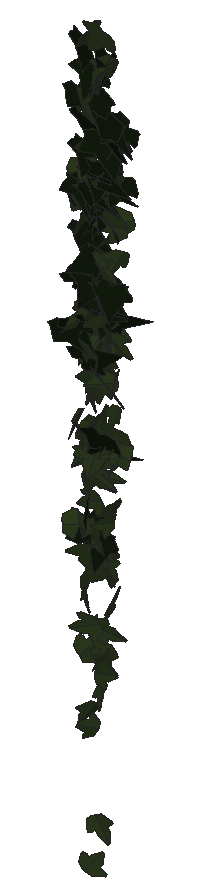
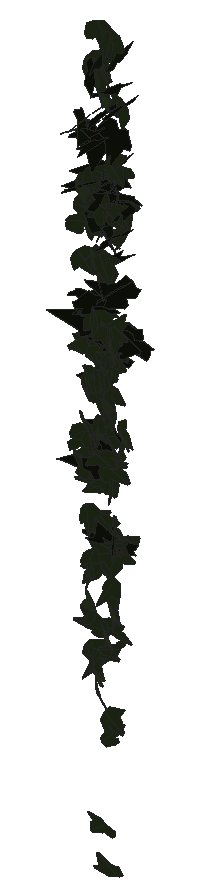
# SketchUp Ruby script. Lengths in inches.
U = 1.inch
M = Sketchup.active_model
def pt(a) = Geom::Point3d.new(a.map { |v| v * U })
def face(e, loops, mat)
  f = e.add_face(loops[0].map { |a| pt(a) })
  loops[1..].each { |l| e.add_face(l.map { |a| pt(a) }).erase! }
  f.material = f.back_material = mat if mat
  f
end
# faces: each face lists its corners as indices into pts; further lists are holes
def faces(e, pts, list, mat = nil) = list.each { |f| face(e, (f[0].is_a?(Array) ? f : [f]).map { |l| l.map { |i| pts[i] } }, mat) }
# xy, xz, yz: faces in a plane at the given z, y or x. An outline is a flat list of corners, or four numbers for a rectangle; further outlines are holes
def ring(l) = l.size == 4 ? [[l[0], l[1]], [l[2], l[1]], [l[2], l[3]], [l[0], l[3]]] : l.each_slice(2).to_a
def flat(e, list, mat, &to3) = list.each { |f| face(e, (f[0].is_a?(Array) ? f : [f]).map { |l| ring(l).map { |u, v| to3.(u, v) } }, mat) }
def xy(e, z, list, mat = nil) = flat(e, list, mat) { |x, y| [x, y, z] }
def xz(e, y, list, mat = nil) = flat(e, list, mat) { |x, z| [x, y, z] }
def yz(e, x, list, mat = nil) = flat(e, list, mat) { |y, z| [x, y, z] }
def lines(e, pts, list) = list.each { |a, b| e.add_line(pt(pts[a]), pt(pts[b])) }
# prism: a flat outline (further loops are holes) pulled along v
def prism(e, loops, v, mat = nil)
  f = face(e, loops, mat); d = Geom::Vector3d.new(v.map { |x| x * U })
  f.pushpull(f.normal.samedirection?(d) ? d.length : -d.length)
end
def box(e, o, s, mat = nil) = prism(e, [[o, [o[0] + s[0], o[1], o[2]], [o[0] + s[0], o[1] + s[1], o[2]], [o[0], o[1] + s[1], o[2]]]], [0, 0, s[2]], mat)
def at(x, y, z, deg = 0) = Geom::Transformation.translation(pt([x, y, z])) * Geom::Transformation.rotation(ORIGIN, Z_AXIS, deg.degrees)
def axes(o, x, y, z) = Geom::Transformation.new([*x, 0, *y, 0, *z, 0, *pt(o).to_a, 1])
def part(name) = M.definitions.add(name)
# library, detail: a bought-in or finely detailed component or shape, given as its bounding box
def library(name, o, s) = part(name).tap { |d| box(d.entities, o, s) }
def detail(e, o, s) = box(e.add_group.entities, o, s)
def put(e, d, t, mat = nil) = e.add_instance(d, t).tap { |i| i.material = mat if mat }
def group(e, t, mat = nil) = e.add_group.tap { |g| g.transformation = t; g.material = mat if mat }.entities
root = M.entities
M.materials.add("1026 AP 7946 SUNNY SIDE UP").color = [254, 231, 186]
M.materials.add("efeu1").color = [18, 25, 13]
M.materials.add("efeu2").color = [43, 57, 29]
c1 = part("ivyleaf_10")
p = [[0,0.5,-0.03],[-0.0625,2.02,-0.43],[-0.19,2.01,-0.46],[-0.54,1.05,-0.29],[-0.52,0.625,-0.18],[-0.83,0.76,-0.28],
  [-1.16,0.64,-0.33],[-1.15,0.33,-0.24],[-0.77,-0.39,0.02],[-0.3,-0.51,0.16],[0.04,-0.48,0.23],[-0.02,2.01,-0.4375],
  [-0.06,2.01,-0.43],[0.04,-0.49,0.23],[0.67,-0.49,0.14],[1.38,0.36,-0.2],[1.375,0.51,-0.24],[0.81,0.65,-0.19],
  [0.62,0.59,-0.15],[0.6,1.09,-0.28],[0.5,1.23,-0.31]]
faces(c1.entities,p,[[0,1,2,3,4,5,6,7,8,9,10],[11,12,0,13,14,15,16,17,18,19,20]],"efeu2")
c2 = part("ivyleaf_9")
p = [[1.54,2.16,1.25],[1.36,2.04,1.19],[-0.21,0.99,0.68],[-0.71,1.11,0.82],[-0.85,0.86,0.67],[-0.8,0.17,0.21],
  [-0.9,-0.01,0.1],[-0.67,-0.16,-0.02],[-0.08,-0.08,-0.05],[-0.03,-0.6,-0.4],[0.65,-0.88,-0.66],[0.83,-0.6,-0.49],
  [1.29,-0.42,-0.43],[1.8125,-0.07,-0.26],[1.21,0.44,0.15]]
faces(c2.entities,p,[[0,1,2,3,4,5,6,7,8,9,10,11,12,13,14]],"efeu1")
put(root,c1,axes([106.17,212.36,258.08],[-0.20733,0.18687,0.08375],[0.07494,-0.06456,0.23523],[0.31087,0.1402,-0.00085]),"1026 AP 7946 SUNNY SIDE UP")
put(root,c1,axes([106.34,212.28,263.92],[-0.33915,-0.0739,0.11531],[-0.15457,-0.05825,-0.23424],[0.14429,-0.23612,0.0201]),"1026 AP 7946 SUNNY SIDE UP")
put(root,c1,axes([106.14,212.3,258.68],[0.16961,-0.19678,0.12508],[0.06388,-0.11701,-0.23111],[0.35886,0.11384,-0.01798]),"1026 AP 7946 SUNNY SIDE UP")
put(root,c1,axes([106.21,212.55,264.98],[0.01795,-0.24608,0.10694],[0.02224,-0.10459,-0.25424],[0.42022,0.01604,0.00889]),"1026 AP 7946 SUNNY SIDE UP")
put(root,c2,axes([105.98,212.14,260.81],[-0.09391,-0.08738,-0.23628],[0.27532,0.14952,-0.10501],[0.2694,-0.18327,0.02496]),"1026 AP 7946 SUNNY SIDE UP")
put(root,c1,axes([106.36,212.21,256.09],[0.2074,-0.01936,0.18283],[-0.26065,0.06899,0.135],[-0.10466,-0.21017,0.0261]),"1026 AP 7946 SUNNY SIDE UP")
put(root,c1,axes([106.22,212.48,260.36],[-0.05254,-0.20434,-0.10501],[0.02558,0.09945,-0.21272],[0.35733,-0.03717,-0.00021]),"1026 AP 7946 SUNNY SIDE UP")
put(root,c1,axes([106,212.17,256.13],[0.08141,-0.06725,-0.23613],[0.29084,0.15915,-0.00414],[0.23677,-0.17237,0.08628]),"1026 AP 7946 SUNNY SIDE UP")
put(root,c1,axes([106.19,212.5,260.3125],[0.04478,0.16939,-0.1684],[-0.04149,-0.1623,-0.1779],[-0.36887,0.03882,-0.00043]),"1026 AP 7946 SUNNY SIDE UP")
put(root,c1,axes([106.22,212.53,254.72],[0.10449,-0.19811,0.05644],[0.0243,-0.05379,-0.21557],[0.32276,0.06818,-0.00204]),"1026 AP 7946 SUNNY SIDE UP")
put(root,c2,axes([106.21,212.36,265.67],[0.35397,-0.0276,-0.15543],[-0.24035,-0.02181,-0.23121],[0.01677,0.27003,-0.03295]),"1026 AP 7946 SUNNY SIDE UP")
put(root,c1,axes([106.32,212.6,263.89],[-0.17824,-0.15521,0.146],[-0.04027,-0.15058,-0.19069],[0.32897,-0.10253,0.05576]),"1026 AP 7946 SUNNY SIDE UP")
put(root,c1,axes([106.26,212.39,261.04],[-0.02348,-0.06015,0.26537],[0.02207,-0.25816,-0.0627],[0.41587,0.0103,0.01831]),"1026 AP 7946 SUNNY SIDE UP")
put(root,c1,axes([106.14,212.5,264.31],[-0.07374,0.08614,-0.22795],[0.08089,-0.217,-0.09932],[-0.36522,-0.06545,0.02403]),"1026 AP 7946 SUNNY SIDE UP")
put(root,c1,axes([106.29,212.1,263.15],[0.04385,-0.04155,0.25671],[-0.13514,0.23444,0.0515],[-0.37393,-0.0896,0.01149]),"1026 AP 7946 SUNNY SIDE UP")
put(root,c1,axes([106.39,212.53,256.66],[0.19892,-0.06102,-0.15531],[-0.21651,0.06065,-0.14429],[0.13517,0.18695,-0.00256]),"1026 AP 7946 SUNNY SIDE UP")
put(root,c2,axes([106.35,212.28,256.49],[0.06178,-0.04328,-0.24801],[-0.31387,0.13482,-0.0578],[0.22163,0.203,-0.01272]),"1026 AP 7946 SUNNY SIDE UP")
put(root,c1,axes([106.36,212.51,261.01],[-0.33357,-0.03615,0.06661],[-0.09204,-0.03942,-0.22007],[0.07186,-0.21831,0.02736]),"1026 AP 7946 SUNNY SIDE UP")
put(root,c2,axes([106,212.13,260.73],[0.16843,0.05581,0.23152],[0.33879,0.06573,-0.12241],[-0.13205,0.23982,-0.01874]),"1026 AP 7946 SUNNY SIDE UP")
put(root,c1,axes([106.25,212.46,260.69],[0.08806,-0.20288,0.09923],[0.05222,-0.0919,-0.21725],[0.35005,0.06475,0.00744]),"1026 AP 7946 SUNNY SIDE UP")
put(root,c1,axes([106.2,212.54,259.17],[-0.18005,0.15457,-0.08059],[0.06462,-0.06793,-0.19844],[-0.26526,-0.12146,0.00635]),"1026 AP 7946 SUNNY SIDE UP")
put(root,c1,axes([106.39,212.41,257.8125],[-0.13486,-0.12628,0.156],[-0.113,-0.13459,-0.15761],[0.28964,-0.11131,0.01114]),"1026 AP 7946 SUNNY SIDE UP")
put(root,c2,axes([106.1,212.35,266.28],[0.12046,-0.25366,-0.08776],[-0.02131,0.08332,-0.27227],[0.41949,0.07708,0.01137]),"1026 AP 7946 SUNNY SIDE UP")
put(root,c1,axes([106.24,212.68,259.55],[0.05685,-0.15964,0.15075],[0.08218,-0.13848,-0.16871],[0.33145,0.06171,0.01597]),"1026 AP 7946 SUNNY SIDE UP")
put(root,c2,axes([106.08,212.29,261.82],[0.00888,-0.00129,0.26076],[0.37397,0.0867,-0.0045],[-0.13625,0.23788,0.00464]),"1026 AP 7946 SUNNY SIDE UP")
put(root,c1,axes([106.37,212.21,254.52],[-0.14827,0.14765,0.13583],[-0.12718,0.10354,-0.17959],[-0.28313,-0.12383,0.00954]),"1026 AP 7946 SUNNY SIDE UP")
put(root,c2,axes([106.16,212.43,267.32],[-0.00258,-0.19972,0.18724],[0.00235,-0.18289,-0.20681],[0.42581,-0.0002,0.00228]),"1026 AP 7946 SUNNY SIDE UP")
put(root,c1,axes([106.29,212.6,259.29],[0.18601,-0.17829,0.03368],[0.01611,-0.03361,-0.22039],[0.28486,0.11832,-0.00953]),"1026 AP 7946 SUNNY SIDE UP")
put(root,c2,axes([106.21,212.45,264.84],[-0.0488,-0.20698,0.13975],[-0.00643,-0.13745,-0.21596],[0.39009,-0.02816,0.01392]),"1026 AP 7946 SUNNY SIDE UP")
put(root,c2,axes([106.29,212.62,266.7],[-0.15011,-0.2225,0.07101],[-0.01559,-0.07191,-0.24912],[0.36652,-0.09419,0.01849]),"1026 AP 7946 SUNNY SIDE UP")
put(root,c1,axes([106.19,212.46,258.29],[0.23853,-0.0907,0.1462],[0.16646,-0.09808,-0.18108],[0.20685,0.18352,-0.02287]),"1026 AP 7946 SUNNY SIDE UP")
put(root,c1,axes([106.36,212.125,260.48],[-0.29982,0.11659,0.00771],[-0.02687,-0.01494,-0.22925],[-0.18167,-0.19021,0.02119]),"1026 AP 7946 SUNNY SIDE UP")
put(root,c1,axes([106.16,212.27,266.16],[-0.17241,0.08051,-0.24277],[0.2305,-0.18789,-0.13723],[-0.31738,-0.18019,0.03221]),"1026 AP 7946 SUNNY SIDE UP")
put(root,c1,axes([106.38,212.36,267.72],[-0.07357,-0.23047,-0.16421],[0.05122,0.1547,-0.24136],[0.43645,-0.05701,0.00064]),"1026 AP 7946 SUNNY SIDE UP")
put(root,c1,axes([106.4375,212.64,258.17],[0.20828,0.11392,-0.13528],[-0.14482,-0.09499,-0.18027],[-0.23274,0.16105,-0.00889]),"1026 AP 7946 SUNNY SIDE UP")
put(root,c1,axes([106.44,212.59,262.68],[-0.10697,-0.21769,0.03991],[-0.00785,-0.0403,-0.23508],[0.34793,-0.06783,0.00697]),"1026 AP 7946 SUNNY SIDE UP")
put(root,c2,axes([106.31,212.35,264.14],[-0.22126,-0.18156,-0.11538],[0.15175,0.06412,-0.23376],[0.29819,-0.16734,0.03335]),"1026 AP 7946 SUNNY SIDE UP")
put(root,c1,axes([106.42,212.52,260.08],[0.01291,-0.21517,-0.06571],[0.01909,0.06294,-0.22099],[0.35182,0.00448,0.0144]),"1026 AP 7946 SUNNY SIDE UP")
put(root,c2,axes([106.37,212.42,261.85],[-0.11322,-0.21238,0.12841],[-0.04726,-0.12258,-0.23153],[0.38529,-0.07744,0.00933]),"1026 AP 7946 SUNNY SIDE UP")
put(root,c2,axes([106.24,212.29,263.19],[0.17485,-0.18056,-0.17361],[-0.04148,0.17399,-0.21024],[0.38503,0.10074,0.05619]),"1026 AP 7946 SUNNY SIDE UP")
put(root,c2,axes([106.4,212.33,263.83],[0.17196,-0.11205,-0.2086],[-0.24119,0.13166,-0.16013],[0.2713,0.18807,-0.01015]),"1026 AP 7946 SUNNY SIDE UP")
put(root,c1,axes([106.375,212.32,255.08],[-0.03474,-0.16013,-0.19442],[0.11748,0.17537,-0.16207],[0.36987,-0.07074,0.03322]),"1026 AP 7946 SUNNY SIDE UP")
put(root,c1,axes([106.49,212.28,251.97],[-0.03873,-0.19817,0.11264],[-0.02551,-0.10929,-0.20635],[0.35583,-0.02941,-0.00254]),"1026 AP 7946 SUNNY SIDE UP")
put(root,c1,axes([106.5,212.09,257.36],[-0.07802,0.15391,0.18517],[-0.14048,0.15692,-0.16372],[-0.34342,-0.09916,0.0249]),"1026 AP 7946 SUNNY SIDE UP")
put(root,c2,axes([106.22,212.36,264.01],[-0.02716,-0.07377,-0.25379],[0.17644,0.21953,-0.07468],[0.36313,-0.11218,0.0173]),"1026 AP 7946 SUNNY SIDE UP")
put(root,c1,axes([106.34,212.23,264.67],[0.31457,0.13701,0.02611],[0.04398,0.00257,-0.24938],[-0.2144,0.20154,-0.01284]),"1026 AP 7946 SUNNY SIDE UP")
put(root,c2,axes([106.41,212.6,263.41],[-0.25216,0.0307,-0.19145],[0.27551,-0.06586,-0.16721],[-0.10941,-0.2366,0.02019]),"1026 AP 7946 SUNNY SIDE UP")
put(root,c1,axes([106.16,212.58,260.33],[-0.00749,-0.01037,0.23903],[0.36441,0.01597,0.00573],[-0.02546,0.23158,0.01168]),"1026 AP 7946 SUNNY SIDE UP")
put(root,c1,axes([106.63,212.15,253.99],[0.19782,-0.0573,-0.17662],[-0.26579,0.03561,-0.1401],[0.09935,0.20938,-0.02316]),"1026 AP 7946 SUNNY SIDE UP")
put(root,c1,axes([106.57,212.53,259.49],[-0.26463,0.10457,0.07881],[-0.1461,-0.01133,-0.19623],[-0.14118,-0.18427,0.05535]),"1026 AP 7946 SUNNY SIDE UP")
put(root,c1,axes([106.375,212.625,266.59],[0.14064,-0.14966,0.1966],[0.14051,-0.16973,-0.18046],[0.35564,0.12624,-0.00645]),"1026 AP 7946 SUNNY SIDE UP")
put(root,c1,axes([106.49,212.37,259.58],[-0.39898,0.01824,-0.00673],[0.00735,-0.027,-0.2608],[-0.02963,-0.25238,0.02592]),"1026 AP 7946 SUNNY SIDE UP")
put(root,c1,axes([106.52,212.43,264.06],[0.16552,-0.13106,-0.17869],[-0.05801,0.17836,-0.16155],[0.33593,0.09538,0.06015]),"1026 AP 7946 SUNNY SIDE UP")
put(root,c2,axes([106.43,212.23,255.89],[-0.32401,0.03737,0.16518],[0.25087,-0.01663,0.21542],[0.06251,0.26043,-0.00839]),"1026 AP 7946 SUNNY SIDE UP")
put(root,c1,axes([106.39,212.35,260.27],[0.17732,0.11369,-0.15923],[0.11591,0.14064,0.16213],[0.27943,-0.13049,0.03379]),"1026 AP 7946 SUNNY SIDE UP")
put(root,c1,axes([106.53,212.2,255.7],[-0.31291,-0.17336,0.00168],[0.01718,-0.01651,-0.27123],[0.27208,-0.19833,0.01906]),"1026 AP 7946 SUNNY SIDE UP")
put(root,c2,axes([106.5625,212.38,262.42],[-0.15697,-0.12815,0.22117],[-0.17755,-0.18401,-0.16776],[0.35186,-0.15002,0.01401]),"1026 AP 7946 SUNNY SIDE UP")
put(root,c1,axes([106.51,212.31,251.47],[-0.00624,0.09865,0.19903],[0.01739,-0.19233,0.10057],[0.33987,0.01165,-0.00149]),"1026 AP 7946 SUNNY SIDE UP")
put(root,c2,axes([106.24,212.36,263.83],[0.24059,-0.17517,0.11175],[0.09539,-0.09212,-0.23975],[0.31048,0.16405,-0.01294]),"1026 AP 7946 SUNNY SIDE UP")
put(root,c1,axes([106.39,212.4,253.73],[0.09725,-0.12721,-0.15696],[0.13129,-0.12727,0.14433],[-0.28217,-0.10306,0.01306]),"1026 AP 7946 SUNNY SIDE UP")
put(root,c2,axes([106.41,212.57,266.12],[0.07787,-0.24413,-0.06587],[-0.03387,0.05942,-0.2561],[0.39482,0.05324,-0.00898]),"1026 AP 7946 SUNNY SIDE UP")
put(root,c1,axes([106.59,212.47,259.74],[-0.0163,-0.19104,0.12763],[0.00136,-0.12513,-0.19772],[0.35896,-0.0082,0.00654]),"1026 AP 7946 SUNNY SIDE UP")
put(root,c1,axes([106.6,212.6,262.77],[0.0614,-0.22971,0.02809],[0.00081,-0.02889,-0.24016],[0.36397,0.03881,-0.0042]),"1026 AP 7946 SUNNY SIDE UP")
put(root,c2,axes([106.46,212.51,264.39],[-0.05821,-0.23811,0.1155],[0.02215,-0.1162,-0.24716],[0.41416,-0.02725,0.02945]),"1026 AP 7946 SUNNY SIDE UP")
put(root,c1,axes([106.77,212.26,267.82],[-0.35601,0.05025,0.13611],[-0.21439,-0.01382,-0.23587],[-0.05706,-0.26163,0.03701]),"1026 AP 7946 SUNNY SIDE UP")
put(root,c1,axes([106.64,212.42,266.82],[0.05518,-0.27743,-0.09139],[-0.01821,0.08636,-0.28758],[0.45688,0.03695,-0.00042]),"1026 AP 7946 SUNNY SIDE UP")
put(root,c1,axes([106.5,211.99,253.4],[0.12518,0.05749,-0.226],[0.1403,0.20617,0.0901],[0.32837,-0.11,0.04766]),"1026 AP 7946 SUNNY SIDE UP")
put(root,c1,axes([106.61,212.48,258.79],[-0.00084,-0.19201,-0.10703],[0.02748,0.10243,-0.19659],[0.34135,-0.00872,0.01557]),"1026 AP 7946 SUNNY SIDE UP")
put(root,c2,axes([106.47,212.09,264.28],[0.24852,-0.13811,-0.15342],[-0.11925,0.13388,-0.21115],[0.29529,0.1703,0.04385]),"1026 AP 7946 SUNNY SIDE UP")
put(root,c1,axes([106.63,212.47,258.77],[0.0501,-0.20321,0.07242],[0.01001,-0.07131,-0.21227],[0.33856,0.03218,-0.00444]),"1026 AP 7946 SUNNY SIDE UP")
put(root,c1,axes([106.625,212.59,259.89],[0.00136,-0.19049,0.10999],[0.02761,-0.10744,-0.19627],[0.34309,0.0094,0.01536]),"1026 AP 7946 SUNNY SIDE UP")
put(root,c1,axes([106.65,212.4,262.2],[0.08522,-0.22582,-0.05665],[-0.01121,0.0535,-0.23887],[0.36482,0.05439,0.00589]),"1026 AP 7946 SUNNY SIDE UP")
put(root,c2,axes([106.81,212.65,261.52],[-0.07745,0.00611,0.25172],[-0.33851,-0.11903,-0.04234],[0.18186,-0.21896,0.02839]),"1026 AP 7946 SUNNY SIDE UP")
put(root,c1,axes([106.59,212.23,257.94],[0.37564,-0.00386,-0.01181],[-0.01845,-0.02079,-0.24531],[0.00448,0.23826,-0.02019]),"1026 AP 7946 SUNNY SIDE UP")
put(root,c2,axes([106.53,212.64,267.17],[-0.07894,-0.13575,0.22304],[0.00442,-0.22168,-0.14332],[0.40282,-0.02417,0.04528]),"1026 AP 7946 SUNNY SIDE UP")
put(root,c2,axes([106.75,212.375,263.59],[-0.15352,0.19218,-0.14327],[0.08688,-0.12904,-0.22268],[-0.36378,-0.11192,0.00728]),"1026 AP 7946 SUNNY SIDE UP")
put(root,c1,axes([106.4,212.32,258.53],[0.16658,0.00113,0.21861],[0.33355,-0.0067,-0.1091],[0.00863,0.23707,-0.00274]),"1026 AP 7946 SUNNY SIDE UP")
put(root,c1,axes([106.45,212.27,256],[0.1813,-0.03816,0.18675],[0.27625,-0.04598,-0.12521],[0.09341,0.21004,0.00785]),"1026 AP 7946 SUNNY SIDE UP")
put(root,c1,axes([106.58,212.45,260.34],[0.10253,-0.12774,0.18836],[0.15412,-0.15554,-0.14828],[0.31606,0.11728,0.01121]),"1026 AP 7946 SUNNY SIDE UP")
put(root,c1,axes([106.69,212.5,261.36],[0.02761,-0.20979,-0.09604],[0.02938,0.09331,-0.2149],[0.35903,0.0085,0.02497]),"1026 AP 7946 SUNNY SIDE UP")
put(root,c2,axes([106.4,212.14,260.125],[-0.0022,0.02724,0.25442],[0.34677,-0.11327,0.01351],[0.1794,0.21928,-0.02299]),"1026 AP 7946 SUNNY SIDE UP")
put(root,c1,axes([106.52,212.37,255.79],[-0.19592,0.02972,-0.16682],[0.22477,-0.08165,-0.12909],[-0.12897,-0.18744,0.02845]),"1026 AP 7946 SUNNY SIDE UP")
put(root,c1,axes([106.48,212.48,260.86],[-0.20299,0.03014,0.19826],[0.3052,0.00291,0.1338],[0.02259,0.23158,-0.02611]),"1026 AP 7946 SUNNY SIDE UP")
put(root,c1,axes([106.54,212.12,248.3],[0.2865,-0.03067,-0.09394],[0.14601,0.0064,0.18932],[-0.03858,-0.20357,0.01888]),"1026 AP 7946 SUNNY SIDE UP")
put(root,c1,axes([106.55,212.29,257.4],[-0.22426,-0.05792,-0.1559],[0.23419,0.03145,-0.15716],[0.09914,-0.20531,0.01858]),"1026 AP 7946 SUNNY SIDE UP")
put(root,c1,axes([106.64,212.47,253.05],[0.11553,-0.13936,0.14741],[0.0997,-0.12919,-0.16302],[0.29876,0.097,-0.0026]),"1026 AP 7946 SUNNY SIDE UP")
put(root,c1,axes([106.61,212.61,259.98],[-0.21649,0.10661,-0.12779],[0.12076,-0.1019,-0.17777],[-0.2279,-0.15527,0.02719]),"1026 AP 7946 SUNNY SIDE UP")
put(root,c1,axes([106.64,212.46,261.34],[-0.29982,-0.08425,-0.08348],[0.13932,-0.00441,-0.21134],[0.1191,-0.20694,0.03708]),"1026 AP 7946 SUNNY SIDE UP")
put(root,c1,axes([106.71,212.6,263.49],[0.01691,-0.18899,0.14969],[0.04586,-0.14439,-0.19511],[0.37306,0.02632,0.0172]),"1026 AP 7946 SUNNY SIDE UP")
put(root,c1,axes([106.51,212.34,262.42],[-0.22342,0.01219,-0.19974],[0.27589,-0.09527,-0.13914],[-0.1314,-0.22075,0.04748]),"1026 AP 7946 SUNNY SIDE UP")
put(root,c2,axes([106.8,212.15,258.48],[0.24761,0.05879,-0.17883],[-0.23981,-0.08567,-0.17259],[-0.16071,0.21842,-0.01799]),"1026 AP 7946 SUNNY SIDE UP")
put(root,c1,axes([106.92,212.27,253.41],[-0.11591,-0.05624,0.20167],[-0.2,-0.15032,-0.09456],[0.25075,-0.14589,0.0178]),"1026 AP 7946 SUNNY SIDE UP")
put(root,c2,axes([106.69,212.69,267.01],[-0.12148,0.03053,-0.25534],[0.2828,-0.17346,-0.08072],[-0.27283,-0.19339,0.03002]),"1026 AP 7946 SUNNY SIDE UP")
put(root,c1,axes([106.79,212.15,261.49],[0.16556,-0.15856,-0.16956],[-0.03464,0.17239,-0.18562],[0.35666,0.09035,0.06068]),"1026 AP 7946 SUNNY SIDE UP")
put(root,c2,axes([106.44,212.22,264.55],[0.06934,-0.06733,-0.25548],[0.31287,0.16762,-0.00947],[0.25477,-0.18751,0.08116]),"1026 AP 7946 SUNNY SIDE UP")
put(root,c1,axes([106.69,212.29,264.23],[-0.10842,-0.18461,-0.16401],[0.1499,0.13069,-0.19921],[0.35162,-0.11264,0.03436]),"1026 AP 7946 SUNNY SIDE UP")
put(root,c1,axes([106.51,212.3,257.49],[-0.09236,-0.03849,-0.23344],[0.35051,0.04652,-0.06746],[0.08665,-0.2292,0.02407]),"1026 AP 7946 SUNNY SIDE UP")
put(root,c2,axes([106.67,212.5,263.62],[-0.04339,-0.18503,0.1671],[-0.02068,-0.16293,-0.19348],[0.38744,-0.02942,0.00838]),"1026 AP 7946 SUNNY SIDE UP")
put(root,c1,axes([106.76,212.3,267.02],[0.2347,-0.21779,0.03567],[0.01084,-0.03867,-0.27173],[0.34689,0.14856,-0.01564]),"1026 AP 7946 SUNNY SIDE UP")
put(root,c1,axes([106.82,212.43,267.09],[-0.07319,-0.19838,0.19236],[0.01263,-0.19147,-0.20738],[0.42941,-0.02818,0.03888]),"1026 AP 7946 SUNNY SIDE UP")
put(root,c1,axes([106.83,212.42,264.49],[-0.08514,-0.23692,-0.01041],[0.0038,0.00843,-0.25032],[0.37277,-0.0542,0.00017]),"1026 AP 7946 SUNNY SIDE UP")
put(root,c2,axes([106.64,212.47,265.33],[0.04192,-0.22539,-0.09775],[0.02603,0.09561,-0.23176],[0.38287,0.01818,0.02646]),"1026 AP 7946 SUNNY SIDE UP")
put(root,c1,axes([106.94,212.33,259.69],[-0.06204,0.01084,0.21533],[-0.15491,-0.18856,-0.01018],[0.29026,-0.09831,0.04059]),"1026 AP 7946 SUNNY SIDE UP")
put(root,c1,axes([106.68,212.36,252.45],[0.19411,-0.10323,0.168],[0.16628,-0.12658,-0.16517],[0.2548,0.16125,-0.0202]),"1026 AP 7946 SUNNY SIDE UP")
put(root,c2,axes([106.82,212.26,265.36],[0.3499,0.00091,-0.17184],[-0.2598,-0.03706,-0.22749],[-0.03609,0.27562,-0.02838]),"1026 AP 7946 SUNNY SIDE UP")
put(root,c2,axes([106.78,212.48,261.375],[-0.21362,-0.19804,-0.02681],[0.03823,0.01348,-0.247],[0.31151,-0.13746,0.01192]),"1026 AP 7946 SUNNY SIDE UP")
put(root,c1,axes([106.83,212.18,261.2],[-0.16003,-0.19924,-0.01733],[0.0374,0.00541,-0.22965],[0.31202,-0.10284,0.01864]),"1026 AP 7946 SUNNY SIDE UP")
put(root,c2,axes([106.8,212.27,256.02],[-0.31535,-0.0375,-0.13993],[0.2152,0.00283,-0.20929],[0.05136,-0.24208,0.01778]),"1026 AP 7946 SUNNY SIDE UP")
put(root,c2,axes([106.5,212.3,264.26],[0.33227,-0.03797,0.14185],[0.20684,-0.04506,-0.22068],[0.08835,0.24828,-0.01682]),"1026 AP 7946 SUNNY SIDE UP")
put(root,c1,axes([106.74,212.37,253.18],[0.02424,-0.03988,0.22033],[0.14261,-0.19396,-0.04508],[0.31134,0.09195,0.00349]),"1026 AP 7946 SUNNY SIDE UP")
put(root,c2,axes([106.57,212.3125,259.83],[0.23676,-0.19254,0.09869],[0.08296,-0.08167,-0.25214],[0.32861,0.15934,-0.00745]),"1026 AP 7946 SUNNY SIDE UP")
put(root,c1,axes([106.77,212.27,255.4],[-0.20072,-0.15645,-0.1155],[0.15674,0.06013,-0.20463],[0.25795,-0.15827,0.03447]),"1026 AP 7946 SUNNY SIDE UP")
put(root,c1,axes([106.87,212.34,255.6],[-0.13505,-0.19818,-0.02052],[0.02585,0.01334,-0.22221],[0.31195,-0.0869,0.00953]),"1026 AP 7946 SUNNY SIDE UP")
put(root,c1,axes([106.92,212.35,256.39],[-0.01031,-0.02524,-0.22616],[-0.15568,-0.19586,0.02512],[-0.31039,0.09907,-0.00509]),"1026 AP 7946 SUNNY SIDE UP")
put(root,c1,axes([106.875,212.5,256.7],[-0.04342,-0.23042,-0.0372],[0.0183,0.03364,-0.23876],[0.36597,-0.02902,0.00753]),"1026 AP 7946 SUNNY SIDE UP")
put(root,c1,axes([106.875,212.375,254.33],[0.13202,-0.14758,0.19862],[-0.10913,0.18182,0.17482],[-0.36693,-0.10717,0.01947]),"1026 AP 7946 SUNNY SIDE UP")
put(root,c2,axes([106.59,212.32,257.85],[0.21776,0.03958,0.20336],[0.29557,0.05962,-0.14799],[-0.1124,0.23345,0.00481]),"1026 AP 7946 SUNNY SIDE UP")
put(root,c1,axes([106.83,212.57,260.72],[0.13368,0.2176,-0.07613],[-0.03996,-0.07074,-0.24107],[-0.35976,0.08871,-0.00151]),"1026 AP 7946 SUNNY SIDE UP")
put(root,c2,axes([106.8125,212.52,261.8],[-0.2207,-0.18389,-0.07516],[0.08498,0.04908,-0.23768],[0.29862,-0.14988,0.01209]),"1026 AP 7946 SUNNY SIDE UP")
put(root,c1,axes([106.86,212.23,260.97],[-0.21824,0.17595,-0.00216],[-0.01398,-0.01095,-0.2305],[-0.27635,-0.1384,0.01336]),"1026 AP 7946 SUNNY SIDE UP")
put(root,c1,axes([106.98,212.41,258.5],[-0.34277,-0.04082,0.06613],[-0.0926,-0.03387,-0.22759],[0.0762,-0.22477,0.0209]),"1026 AP 7946 SUNNY SIDE UP")
put(root,c1,axes([106.67,212.23,249.37],[0.25485,0.00398,0.14982],[0.22771,-0.02482,-0.16575],[0.02144,0.21632,-0.0205]),"1026 AP 7946 SUNNY SIDE UP")
put(root,c1,axes([106.86,212.61,258.85],[0.23838,-0.15116,0.03137],[0.01383,-0.03535,-0.21992],[0.24233,0.15071,-0.01831]),"1026 AP 7946 SUNNY SIDE UP")
put(root,c1,axes([107.02,212.51,257.96],[0.17927,0.06859,-0.17475],[-0.22928,-0.08744,-0.13758],[-0.17473,0.1851,0.00124]),"1026 AP 7946 SUNNY SIDE UP")
put(root,c1,axes([106.93,212.29,255.27],[-0.0996,0.18122,0.1061],[-0.07973,0.08991,-0.19654],[-0.31708,-0.07953,0.0161]),"1026 AP 7946 SUNNY SIDE UP")
put(root,c1,axes([106.92,212.15,253.33],[-0.05573,-0.18666,-0.12873],[0.04469,0.12068,-0.19497],[0.34943,-0.0452,0.00441]),"1026 AP 7946 SUNNY SIDE UP")
put(root,c1,axes([106.85,212.63,259.68],[0.13886,-0.1373,0.15416],[0.12716,-0.12683,-0.16892],[0.2939,0.11974,0.00025]),"1026 AP 7946 SUNNY SIDE UP")
put(root,c1,axes([106.9375,212.01,253],[-0.01868,0.0985,0.23364],[-0.04778,0.22418,-0.10089],[-0.38502,-0.0326,0.00119]),"1026 AP 7946 SUNNY SIDE UP")
put(root,c2,axes([106.85,212.29,265.39],[-0.14132,-0.23625,-0.12512],[0.076,0.1101,-0.2597],[0.40975,-0.1019,0.00501]),"1026 AP 7946 SUNNY SIDE UP")
put(root,c2,axes([106.93,212.74,264.3],[-0.16849,-0.21198,0.07141],[-0.00393,-0.07707,-0.24302],[0.35125,-0.10254,0.03154]),"1026 AP 7946 SUNNY SIDE UP")
put(root,c1,axes([106.97,212.59,264.29],[0.05693,-0.19516,0.14638],[0.02853,-0.1422,-0.2052],[0.37954,0.03996,-0.00653]),"1026 AP 7946 SUNNY SIDE UP")
put(root,c1,axes([107.1,212.64,263.39],[-0.10401,0.01759,0.2346],[-0.12972,-0.22281,-0.00827],[0.33472,-0.08089,0.0697]),"1026 AP 7946 SUNNY SIDE UP")
put(root,c1,axes([106.78,212.53,260.59],[-0.21198,0.01071,-0.18093],[0.2613,-0.06519,-0.13584],[-0.09121,-0.21164,0.03132]),"1026 AP 7946 SUNNY SIDE UP")
put(root,c1,axes([107.25,212.18,263.51],[0.065,-0.01818,-0.25494],[-0.38438,0.03948,-0.04484],[0.06604,0.24767,-0.01007]),"1026 AP 7946 SUNNY SIDE UP")
put(root,c1,axes([107.02,212.53,262.59],[-0.12566,-0.19088,0.11993],[0.00811,-0.12628,-0.20846],[0.35236,-0.06517,0.04757]),"1026 AP 7946 SUNNY SIDE UP")
put(root,c2,axes([106.87,212.56,263.6],[0.01293,-0.227,0.08431],[0.00082,-0.08316,-0.23449],[0.38012,0.0079,-0.00236]),"1026 AP 7946 SUNNY SIDE UP")
put(root,c1,axes([107.03,212.17,258.14],[0.11006,-0.20548,-0.03347],[-0.03226,0.02606,-0.2232],[0.32524,0.07212,-0.01081]),"1026 AP 7946 SUNNY SIDE UP")
put(root,c1,axes([106.93,212.47,257.625],[0.10477,-0.22292,0.05136],[0.01196,0.05538,0.23888],[-0.35942,-0.06314,0.02292]),"1026 AP 7946 SUNNY SIDE UP")
put(root,c1,axes([106.74,212.22,253.9],[0.00551,0.02521,0.22824],[0.34436,0.04052,-0.00809],[-0.06474,0.2177,-0.02359]),"1026 AP 7946 SUNNY SIDE UP")
put(root,c2,axes([106.72,212.39,261.04],[0.13641,0.03179,0.24653],[0.37718,0.01557,-0.09169],[-0.04021,0.2539,-0.02374]),"1026 AP 7946 SUNNY SIDE UP")
put(root,c2,axes([107.07,212.71,265.55],[-0.23373,-0.13479,0.15208],[-0.05568,-0.16416,-0.19114],[0.31026,-0.13101,0.08026]),"1026 AP 7946 SUNNY SIDE UP")
put(root,c1,axes([107.13,212.46,258.26],[0.17772,0.08048,-0.18461],[-0.20032,-0.12803,-0.1424],[-0.23599,0.16929,-0.01816]),"1026 AP 7946 SUNNY SIDE UP")
put(root,c2,axes([107.22,212.15,265.46],[-0.1389,0.08561,-0.25749],[-0.28038,0.17584,0.12775],[0.30752,0.19899,0.00017]),"1026 AP 7946 SUNNY SIDE UP")
put(root,c2,axes([106.91,212.29,265.81],[0.1583,-0.22002,-0.09434],[-0.03654,0.08852,-0.24829],[0.37219,0.10227,0.01575]),"1026 AP 7946 SUNNY SIDE UP")
